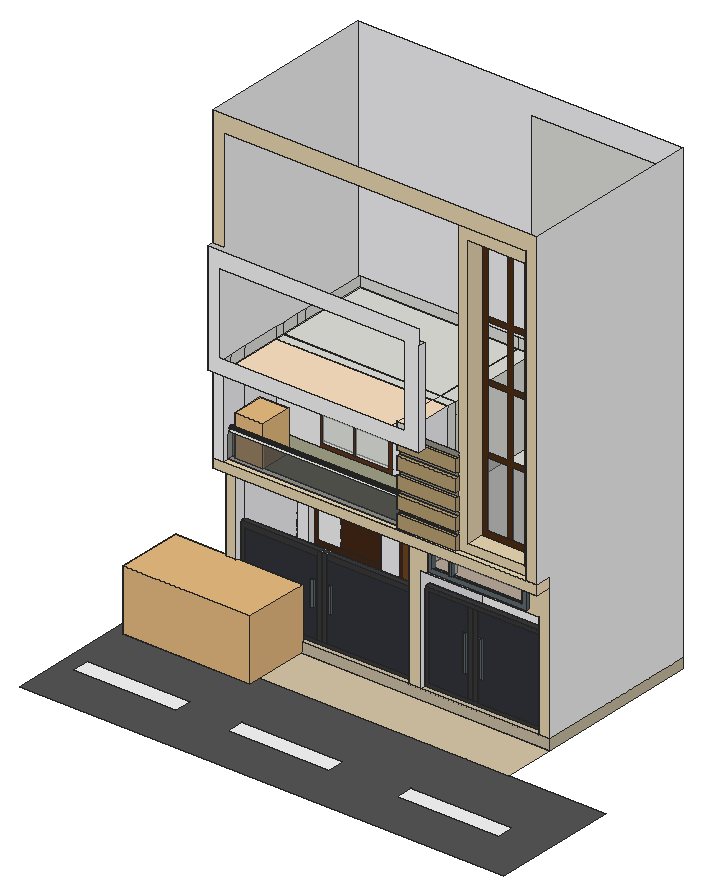
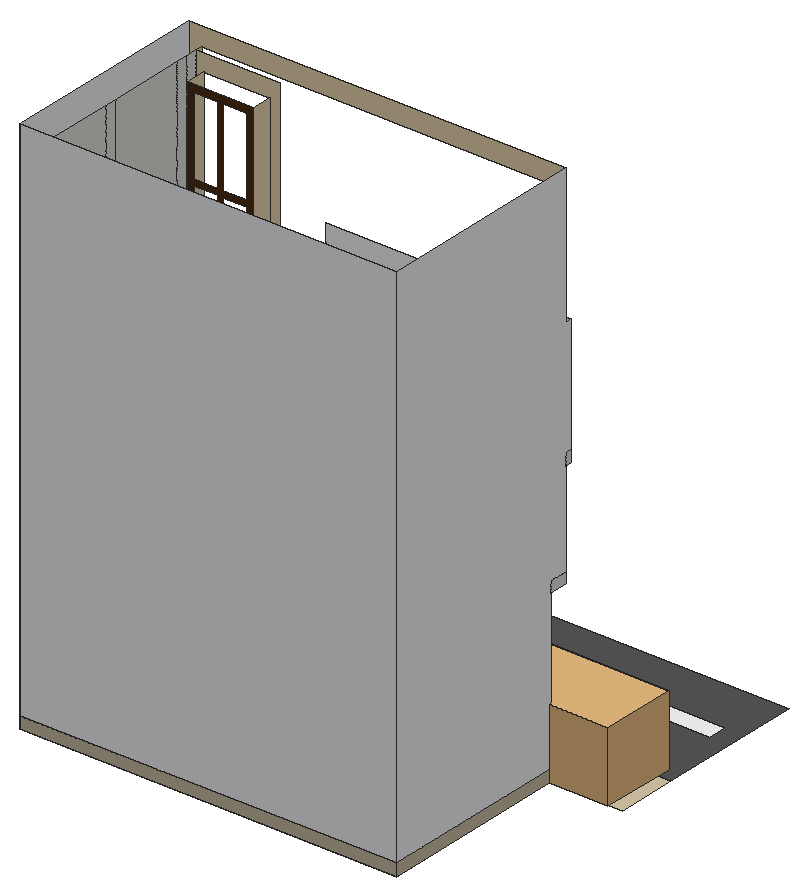
# SketchUp Ruby script. Lengths in inches.
U = 1.inch
M = Sketchup.active_model
def pt(a) = Geom::Point3d.new(a.map { |v| v * U })
def face(e, loops, mat)
  f = e.add_face(loops[0].map { |a| pt(a) })
  loops[1..].each { |l| e.add_face(l.map { |a| pt(a) }).erase! }
  f.material = f.back_material = mat if mat
  f
end
# faces: each face lists its corners as indices into pts; further lists are holes
def faces(e, pts, list, mat = nil) = list.each { |f| face(e, (f[0].is_a?(Array) ? f : [f]).map { |l| l.map { |i| pts[i] } }, mat) }
# xy, xz, yz: faces in a plane at the given z, y or x. An outline is a flat list of corners, or four numbers for a rectangle; further outlines are holes
def ring(l) = l.size == 4 ? [[l[0], l[1]], [l[2], l[1]], [l[2], l[3]], [l[0], l[3]]] : l.each_slice(2).to_a
def flat(e, list, mat, &to3) = list.each { |f| face(e, (f[0].is_a?(Array) ? f : [f]).map { |l| ring(l).map { |u, v| to3.(u, v) } }, mat) }
def xy(e, z, list, mat = nil) = flat(e, list, mat) { |x, y| [x, y, z] }
def xz(e, y, list, mat = nil) = flat(e, list, mat) { |x, z| [x, y, z] }
def yz(e, x, list, mat = nil) = flat(e, list, mat) { |y, z| [x, y, z] }
def lines(e, pts, list) = list.each { |a, b| e.add_line(pt(pts[a]), pt(pts[b])) }
# prism: a flat outline (further loops are holes) pulled along v
def prism(e, loops, v, mat = nil)
  f = face(e, loops, mat); d = Geom::Vector3d.new(v.map { |x| x * U })
  f.pushpull(f.normal.samedirection?(d) ? d.length : -d.length)
end
def box(e, o, s, mat = nil) = prism(e, [[o, [o[0] + s[0], o[1], o[2]], [o[0] + s[0], o[1] + s[1], o[2]], [o[0], o[1] + s[1], o[2]]]], [0, 0, s[2]], mat)
def at(x, y, z, deg = 0) = Geom::Transformation.translation(pt([x, y, z])) * Geom::Transformation.rotation(ORIGIN, Z_AXIS, deg.degrees)
def axes(o, x, y, z) = Geom::Transformation.new([*x, 0, *y, 0, *z, 0, *pt(o).to_a, 1])
def part(name) = M.definitions.add(name)
# library, detail: a bought-in or finely detailed component or shape, given as its bounding box
def library(name, o, s) = part(name).tap { |d| box(d.entities, o, s) }
def detail(e, o, s) = box(e.add_group.entities, o, s)
def put(e, d, t, mat = nil) = e.add_instance(d, t).tap { |i| i.material = mat if mat }
def group(e, t, mat = nil) = e.add_group.tap { |g| g.transformation = t; g.material = mat if mat }.entities
root = M.entities
M.materials.add("[0012_Bisque]").color = [255, 228, 196]
M.materials.add("[Blinds Vertical Pattern]").color = [247, 247, 249]
M.materials.add("[Blinds Vertical Pattern]1").color = [245, 245, 247]
M.materials.add("[Carpet Pattern Squares Multi]").color = [138, 129, 101]
M.materials.add("[Color M06]").color = [86, 86, 86]
M.materials.add("[Color M07]").color = [58, 58, 58]
M.materials.add("[Concrete Tile]").color = [203, 190, 164]
M.materials.add("[Fabric Linen]").color = [161, 161, 136]
M.materials.add("[Field Square Tile]").color = [217, 201, 169]
M.materials.add("[Formica Graystone]").color = [149, 146, 135]
M.materials.add("[Formica Laminate Dark]").color = [50, 53, 60]
M.materials.add("[Formica Speckled Grey]").color = [94, 105, 111]
M.materials.add("[Quartz Light Brown]").color = [234, 216, 179]
M.materials.add("[Quartz Light Grey]").color = [251, 251, 252]
M.materials.add("[Translucent Glass Gray]1").color = [68, 68, 68]
M.materials["[Translucent Glass Gray]1"].alpha = 0.5
M.materials.add("[Translucent Glass Gray]2").color = [128, 128, 128]
M.materials["[Translucent Glass Gray]2"].alpha = 0.5
M.materials.add("[Translucent Glass Safety]1").color = [237, 244, 239]
M.materials["[Translucent Glass Safety]1"].alpha = 0.5
M.materials.add("[Wood Bamboo]").color = [79, 46, 19]
M.materials.add("[Wood Cherry Original]").color = [94, 53, 26]
M.materials.add("[Wood Floor Light]").color = [186, 160, 115]
M.materials.add("[Wood Floor Parquet]").color = [112, 68, 30]
M.materials.add("[Wood Veneer 01]").color = [68, 40, 21]
c1 = library("2015 Porsche Macan",[0.14,0.6,0.32],[90.05,184.43,65.58])
c2 = library("chau cay",[-24.34,-109.24,0],[56.46,62.58,79.69])
xy(root,0,[[123.03,353.85,764.83,681.5]])
xy(root,0,[[[0,0,957,250.875],[33.02,92,234.33,126.875],[336.46,92,537.77,126.875],[671.58,92,872.89,126.875]]],"[Color M06]")
xy(root,0,[[0,250.875,764.83,353.85]],"[Field Square Tile]")
xy(root,0,[[33.02,92,234.33,126.875],[336.46,92,537.77,126.875],[671.58,92,872.89,126.875]],"[Quartz Light Grey]")
xy(root,20.125,[[123.03,353.85,123.03,681.5,764.83,681.5,764.83,353.85,743.35,353.85,743.35,660.02,144.51,660.02,144.51,353.85],[484.74,353.85,509.12,504.41],[144.51,364.59,484.74,375.33],[509.12,364.59,743.35,375.33],[509.12,375.33,743.35,504.41],
  [144.51,504.41,743.35,525.85],[144.51,525.85,743.35,660.02]])
xy(root,20.125,[[144.51,375.33,484.74,504.41]],"[Carpet Pattern Squares Multi]")
xy(root,20.125,[[144.51,353.85,484.74,364.59],[509.12,353.85,743.35,364.59]],"[Concrete Tile]")
xy(root,26.25,[[152.57,364.59,294.93,375.33],[294.93,364.59,304.83,375.33],[304.83,364.59,314.73,375.33],[314.73,364.59,476.37,375.33]])
xy(root,27,[[515.75,364.59,593.81,375.33],[593.81,364.59,603.98,375.33],[603.98,364.59,614.15,375.33],[614.15,364.59,736.66,375.33]])
xy(root,71.5625,[[585.06,361.78,591.37,364.59],[617.68,361.78,623.99,364.59]],"[Formica Speckled Grey]")
xy(root,82.64,[[284.34,361.84,290.96,364.59],[318.96,361.84,325.59,364.59]],"[Formica Speckled Grey]")
xy(root,86.22,[[167.79,504.41,310.48,515.91]],"[Blinds Vertical Pattern]1")
xy(root,132.08,[[284.34,361.84,290.96,364.59],[318.96,361.84,325.59,364.59]],"[Formica Speckled Grey]")
xy(root,142.75,[[585.06,361.78,591.37,364.59],[617.68,361.78,623.99,364.59]],"[Formica Speckled Grey]")
xy(root,185.51,[[144.51,364.59,304.83,375.33],[304.83,364.59,314.73,375.33],[314.73,364.59,476.37,375.33],[476.37,364.59,484.74,375.33]],"[Color M07]")
xy(root,189.34,[[603.98,364.59,614.15,375.33]])
xy(root,197.4375,[[509.12,364.59,736.66,375.33],[736.66,364.59,743.35,375.33]],"[Color M07]")
xy(root,228.92,[[509.12,353.85,743.35,504.41]],"[0012_Bisque]")
xy(root,234.04,[[167.79,504.41,310.48,515.91]],"[Blinds Vertical Pattern]1")
xy(root,235.2,[[527.72,348.16,722.47,353.85]],"[Formica Speckled Grey]")
xy(root,243.53,[[569.36,348.16,574.76,353.85],[569.36,353.85,574.76,361.85]])
xy(root,243.53,[[536.05,348.16,569.36,353.85],[574.76,348.16,714.14,353.85]],"[Formica Speckled Grey]")
xy(root,271.06,[[569.36,348.16,574.76,353.85],[569.36,353.85,574.76,361.85]])
xy(root,271.06,[[536.05,348.16,569.36,353.85],[574.76,348.16,714.14,353.85]],"[Formica Speckled Grey]")
xy(root,279.39,[[527.72,348.16,722.47,353.85]],"[Formica Speckled Grey]")
xy(root,288.25,[[484.74,321.91,509.12,353.85],[509.12,321.91,764.83,353.85],[484.74,353.85,509.12,504.41],[509.12,353.85,743.35,504.41],[144.51,504.41,743.35,525.85],
  [144.51,525.85,743.35,660.02]])
xy(root,288.25,[[123.03,321.91,123.03,353.85,144.51,353.85,144.51,504.41,484.74,504.41,484.74,321.91]],"[0012_Bisque]")
xy(root,307.6875,[[123.03,321.91,144.51,353.85],[743.35,321.91,764.83,353.85],[484.74,326.3,600.81,332.93],[144.51,332.93,484.74,343.39],[484.74,332.93,743.35,660.02],
  [144.51,452.16,484.74,470.45],[144.51,470.45,455.26,660.02],[455.26,470.45,484.74,660.02]])
xy(root,307.6875,[[144.51,343.39,484.74,452.16]],"[Fabric Linen]")
xy(root,307.6875,[[144.51,321.91,484.74,332.93],[484.74,321.91,743.35,321.91,743.35,332.93,600.81,332.93,600.81,326.3,484.74,326.3]],"[Quartz Light Brown]")
xy(root,324.17,[[618.4,332.93,730.9,367.24]],"[Quartz Light Brown]")
xy(root,332.625,[[484.74,326.3,600.81,332.93]],"[Wood Floor Light]")
xy(root,342.125,[[484.74,326.3,600.81,332.93]],"[Wood Floor Light]")
xy(root,357.5625,[[144.51,332.93,484.74,343.39]])
xy(root,367.0625,[[484.74,326.3,600.81,332.93]],"[Wood Floor Light]")
xy(root,376.5625,[[484.74,326.3,600.81,332.93]],"[Wood Floor Light]")
xy(root,401.5,[[484.74,326.3,600.81,332.93]],"[Wood Floor Light]")
xy(root,411,[[484.74,326.3,600.81,332.93]],"[Wood Floor Light]")
xy(root,435.9375,[[484.74,326.3,600.81,332.93]],"[Wood Floor Light]")
xy(root,445.4375,[[484.74,326.3,600.81,332.93]],"[Wood Floor Light]")
xy(root,468.25,[[144.51,452.16,455.26,470.45],[455.26,452.16,484.74,470.45],[144.51,470.45,455.26,660.02],[455.26,470.45,484.74,660.02]])
xy(root,468.25,[[123.03,309.6,123.03,321.91,144.51,321.91,144.51,452.16,455.26,452.16,455.26,309.6],[455.26,309.6,455.26,452.16,484.74,452.16,484.74,324.41,541.38,324.41,541.38,309.6]],"[0012_Bisque]")
xy(root,470.375,[[484.74,326.3,600.81,332.93]],"[Wood Floor Light]")
xz(root,309.6,[[[123.03,468.25,541.38,687.5],[144.51,496.8125,513.0625,656.64]]],"[Blinds Vertical Pattern]")
xz(root,321.91,[[123.03,468.25,144.51,488.6875]])
xz(root,321.91,[[123.03,307.6875,144.51,468.25]],"[Blinds Vertical Pattern]")
xz(root,321.91,[[123.03,288.25,764.83,307.6875],[743.35,307.6875,764.83,307.6875,764.83,923.6875,123.03,923.6875,123.03,687.5,144.51,687.5,144.51,890.6875,743.35,890.6875]],"[Quartz Light Brown]")
xz(root,324.41,[[484.74,468.25,484.74,496.8125,513.0625,496.8125,513.0625,656.64,541.38,656.64,541.38,468.25]])
xz(root,326.3,[[484.74,307.6875,600.81,332.625],[484.74,342.125,600.81,367.0625],[484.74,376.5625,600.81,401.5],[484.74,411,600.81,435.9375],[484.74,445.4375,600.81,470.375]],"[Wood Floor Light]")
xz(root,332.93,[[484.74,307.6875,600.81,332.625],[484.74,342.125,600.81,367.0625],[484.74,376.5625,600.81,401.5],[484.74,411,600.81,435.9375],[484.74,445.4375,600.81,470.375]])
xz(root,332.93,[[484.74,332.625,600.81,342.125],[484.74,367.0625,600.81,376.5625],[484.74,401.5,600.81,411],[484.74,435.9375,600.81,445.4375],[484.74,470.375,600.81,479.875]],"[Formica Graystone]")
xz(root,332.93,[[[600.81,307.6875,743.35,890.6875],[618.4,324.17,730.9,861.54]]],"[Quartz Light Brown]")
xz(root,332.93,[[144.51,307.6875,484.74,357.5625]],"[Translucent Glass Gray]1")
xz(root,343.39,[[144.51,307.6875,484.74,357.5625]],"[Translucent Glass Gray]1")
xz(root,348.16,[[[527.72,235.2,722.47,279.39],[536.05,243.53,714.14,271.06]],[569.36,243.53,574.76,271.06]],"[Formica Speckled Grey]")
xz(root,353.85,[[[527.72,235.2,722.47,279.39],[536.05,243.53,714.14,271.06]],[569.36,243.53,574.76,271.06],[123.03,288.25,144.51,307.6875],[743.35,288.25,764.83,307.6875]])
xz(root,353.85,[[123.03,0,764.83,20.125]],"[Concrete Tile]")
xz(root,353.85,[[123.03,20.125,144.51,288.25],[[484.74,20.125,509.12,20.125,509.12,228.92,743.35,228.92,743.35,20.125,764.83,20.125,764.83,288.25,484.74,288.25],[527.72,235.2,722.47,279.39]]],"[Quartz Light Brown]")
xz(root,353.85,[[536.05,243.53,569.36,271.06],[574.76,243.53,714.14,271.06]],"[Translucent Glass Gray]2")
xz(root,361.78,[[585.06,71.5625,591.37,142.75],[617.68,71.5625,623.99,142.75]],"[Formica Speckled Grey]")
xz(root,361.84,[[284.34,82.64,290.96,132.08],[318.96,82.64,325.59,132.08]],"[Formica Speckled Grey]")
xz(root,361.85,[[569.36,243.53,574.76,271.06]])
xz(root,364.59,[[585.06,71.5625,591.37,142.75],[617.68,71.5625,623.99,142.75]])
xz(root,364.59,[[144.51,20.125,484.74,20.125,484.74,185.51,314.73,185.51,314.73,174.95,476.37,174.95,476.37,26.25,152.57,26.25,152.57,174.95,294.93,174.95,294.93,185.51,144.51,185.51],[[509.12,20.125,743.35,197.4375],[515.75,27,736.66,189.34]],[294.93,26.25,304.83,185.51],[304.83,26.25,314.73,185.51],[593.81,27,603.98,189.34],
  [603.98,27,614.15,189.34]],"[Color M07]")
xz(root,364.59,[[[152.57,26.25,294.93,174.95],[284.34,82.64,290.96,132.08]],[[314.73,26.25,476.37,174.95],[318.96,82.64,325.59,132.08]],[[515.75,27,593.81,189.34],[585.06,71.5625,591.37,142.75]],[[614.15,27,736.66,189.34],[617.68,71.5625,623.99,142.75]]],"[Formica Laminate Dark]")
xz(root,367.24,[[630.125,335.89,670.08,465.11],[679.79,335.89,719.18,465.11]],"[Translucent Glass Gray]2")
xz(root,367.24,[[[618.4,324.17,730.9,861.54],[630.125,335.89,719.18,849.82]],[670.08,335.89,679.79,335.89,679.79,465.11,719.18,465.11,719.18,475.62,679.79,475.62,679.79,594.34,719.18,594.34,719.18,604.84,679.79,604.84,679.79,706.4,719.18,706.4,719.18,716.91,679.79,716.91,679.79,849.82,670.08,849.82,670.08,716.91,630.125,716.91,630.125,706.4,670.08,706.4,670.08,604.84,630.125,604.84,630.125,594.34,670.08,594.34,670.08,475.62,630.125,475.62,630.125,465.11,670.08,465.11]],"[Wood Bamboo]")
xz(root,375.33,[[144.51,20.125,144.51,185.51,294.93,185.51,294.93,174.95,152.57,174.95,152.57,26.25,476.37,26.25,476.37,174.95,314.73,174.95,314.73,185.51,484.74,185.51,484.74,20.125],[[509.12,20.125,743.35,197.4375],[515.75,27,736.66,189.34]],[152.57,26.25,294.93,174.95],[294.93,26.25,304.83,185.51],[304.83,26.25,314.73,185.51],
  [314.73,26.25,476.37,174.95],[515.75,27,593.81,189.34],[593.81,27,603.98,189.34],[603.98,27,614.15,189.34],[614.15,27,736.66,189.34]])
xz(root,452.16,[[144.51,307.6875,230.97,307.6875,230.97,451.25,374.53,451.25,374.53,307.6875,484.74,307.6875,484.74,468.25,144.51,468.25]],"[Blinds Vertical Pattern]")
xz(root,452.16,[[237.93,314.65,297.34,444.29],[302.89,314.65,367.58,444.29]],"[Translucent Glass Safety]1")
xz(root,452.16,[[[230.97,307.6875,374.53,451.25],[237.93,314.65,367.58,444.29]],[297.34,314.65,302.89,444.29]],"[Wood Cherry Original]")
xz(root,470.45,[[144.51,307.6875,455.26,468.25],[455.26,307.6875,484.74,468.25]])
xz(root,504.41,[[484.74,20.125,509.12,288.25],[509.12,228.92,743.35,288.25]])
xz(root,504.41,[[509.12,20.125,743.35,228.92]],"[Blinds Vertical Pattern]")
xz(root,504.41,[[[144.51,20.125,345.37,20.125,345.37,232.5625,467.37,232.5625,467.37,20.125,484.74,20.125,484.74,288.25,144.51,288.25],[167.79,86.22,310.48,234.04]]],"[Blinds Vertical Pattern]1")
xz(root,504.41,[[353.53,28.29,459.21,224.4]],"[Wood Floor Parquet]")
xz(root,504.41,[[[345.37,20.125,467.37,232.5625],[353.53,28.29,459.21,224.4]]],"[Wood Veneer 01]")
xz(root,515.91,[[176.27,94.7,222.36,225.56]],"[Blinds Vertical Pattern]")
xz(root,515.91,[[[167.79,86.22,310.48,234.04],[176.27,94.7,302,225.56]],[222.36,94.7,302,225.56]],"[Wood Veneer 01]")
xz(root,525.85,[[144.51,20.125,743.35,288.25]])
xz(root,660.02,[[144.51,20.125,743.35,288.25],[144.51,288.25,743.35,307.6875],[144.51,307.6875,455.26,468.25],[455.26,307.6875,484.74,468.25],[484.74,307.6875,743.35,890.6875],
  [144.51,468.25,455.26,488.6875],[455.26,468.25,484.74,488.6875]])
xz(root,681.5,[[123.03,20.125,764.83,923.6875]],"[Blinds Vertical Pattern]1")
xz(root,681.5,[[123.03,0,764.83,20.125]],"[Concrete Tile]")
yz(root,123.03,[[321.91,288.25,353.85,307.6875],[309.6,468.25,321.91,488.6875]])
yz(root,123.03,[[353.85,20.125,353.85,307.6875,321.91,307.6875,321.91,488.6875,309.6,488.6875,309.6,687.5,321.91,687.5,321.91,923.6875,681.5,923.6875,681.5,20.125]],"[Blinds Vertical Pattern]1")
yz(root,123.03,[[353.85,0,681.5,20.125]],"[Concrete Tile]")
yz(root,144.51,[[364.59,20.125,375.33,185.51],[504.41,20.125,525.85,288.25],[525.85,20.125,660.02,288.25],[353.85,288.25,375.33,307.6875],[375.33,288.25,504.41,307.6875],
  [504.41,288.25,525.85,307.6875],[525.85,288.25,660.02,307.6875],[332.93,307.6875,343.39,357.5625],[452.16,307.6875,470.45,468.25],[470.45,307.6875,660.02,468.25],
  [338.0625,360.22,337.37,360.31,336.72,360.58,336.16,361,335.74,361.5625,335.47,362.21,335.375,362.91,335.47,363.6,335.74,364.25,336.16,364.81,336.72,365.23,337.37,365.5,338.0625,365.59,338.76,365.5,339.41,365.23,339.96,364.81,340.39,364.25,340.66,363.6,340.75,362.91,340.66,362.21,340.39,361.5625,339.96,361,339.41,360.58,338.76,360.31],[321.91,468.25,321.91,488.6875,341.61,488.6875,332.93,468.25],[332.93,468.25,341.61,488.6875,375.33,488.6875,375.33,468.25],[375.33,468.25,452.16,488.6875],[452.16,468.25,470.45,488.6875],
  [470.45,468.25,504.41,488.6875],[504.41,468.25,525.85,488.6875],[525.85,468.25,660.02,488.6875]])
yz(root,144.51,[[353.85,20.125,364.59,20.125,364.59,185.51,375.33,185.51,375.33,288.25,353.85,288.25],[375.33,20.125,504.41,288.25],[[321.91,307.6875,332.93,307.6875,332.93,357.5625,343.39,357.5625,343.39,307.6875,375.33,307.6875,375.33,468.25,321.91,468.25],[338.0625,360.22,337.37,360.31,336.72,360.58,336.16,361,335.74,361.5625,335.47,362.21,335.375,362.91,335.47,363.6,335.74,364.25,336.16,364.81,336.72,365.23,337.37,365.5,338.0625,365.59,338.76,365.5,339.41,365.23,339.96,364.81,340.39,364.25,340.66,363.6,340.75,362.91,340.66,362.21,340.39,361.5625,339.96,361,339.41,360.58,338.76,360.31]],[375.33,307.6875,452.16,468.25]],"[Blinds Vertical Pattern]")
yz(root,152.57,[[364.59,26.25,375.33,174.95]])
yz(root,167.79,[[504.41,86.22,515.91,234.04]],"[Blinds Vertical Pattern]1")
yz(root,284.34,[[361.84,82.64,364.59,132.08]],"[Formica Speckled Grey]")
yz(root,290.96,[[361.84,82.64,364.59,132.08]],"[Formica Speckled Grey]")
yz(root,294.93,[[364.59,26.25,375.33,174.95]])
yz(root,304.83,[[364.59,26.25,375.33,185.51]])
yz(root,310.48,[[504.41,86.22,515.91,234.04]],"[Blinds Vertical Pattern]1")
yz(root,314.73,[[364.59,26.25,375.33,174.95],[364.59,174.95,375.33,185.51]])
yz(root,318.96,[[361.84,82.64,364.59,132.08]],"[Formica Speckled Grey]")
yz(root,325.59,[[361.84,82.64,364.59,132.08]],"[Formica Speckled Grey]")
yz(root,455.26,[[470.45,307.6875,660.02,468.25]])
yz(root,476.37,[[364.59,26.25,375.33,174.95]])
yz(root,484.74,[[364.59,20.125,375.33,185.51],[332.93,307.6875,343.39,357.5625],[452.16,307.6875,470.45,468.25],[470.45,307.6875,660.02,468.25],[324.41,468.25,326.3,468.25,326.3,470.375,332.93,470.375,332.93,479.875,326.3,479.875,326.3,496.8125,324.41,496.8125],
  [326.3,468.25,332.93,470.375]])
yz(root,484.74,[[353.85,20.125,353.85,288.25,504.41,288.25,504.41,20.125,375.33,20.125,375.33,185.51,364.59,185.51,364.59,20.125],[[343.39,307.6875,343.39,357.5625,332.93,357.5625,332.93,468.25,452.16,468.25,452.16,307.6875],[338.0625,360.22,338.76,360.31,339.41,360.58,339.96,361,340.39,361.5625,340.66,362.21,340.75,362.91,340.66,363.6,340.39,364.25,339.96,364.81,339.41,365.23,338.76,365.5,338.0625,365.59,337.37,365.5,336.72,365.23,336.16,364.81,335.74,364.25,335.47,363.6,335.375,362.91,335.47,362.21,335.74,361.5625,336.16,361,336.72,360.58,337.37,360.31]]],"[Blinds Vertical Pattern]")
yz(root,484.74,[[326.3,307.6875,332.93,332.625],[326.3,342.125,332.93,357.5625],[326.3,357.5625,332.93,367.0625],[326.3,376.5625,332.93,401.5],[326.3,411,332.93,435.9375],
  [326.3,445.4375,332.93,468.25]],"[Wood Floor Light]")
yz(root,509.12,[[364.59,20.125,375.33,197.4375]])
yz(root,509.12,[[353.85,20.125,364.59,20.125,364.59,197.4375,375.33,197.4375,375.33,20.125,504.41,20.125,504.41,228.92,353.85,228.92]],"[Blinds Vertical Pattern]")
yz(root,515.75,[[364.59,27,375.33,189.34]])
yz(root,527.72,[[348.16,235.2,353.85,279.39]],"[Formica Speckled Grey]")
yz(root,536.05,[[348.16,243.53,353.85,271.06]],"[Formica Speckled Grey]")
yz(root,541.38,[[309.6,468.25,324.41,656.64]],"[Blinds Vertical Pattern]")
yz(root,569.36,[[353.85,243.53,361.85,271.06]])
yz(root,569.36,[[348.16,243.53,353.85,271.06]],"[Formica Speckled Grey]")
yz(root,574.76,[[353.85,243.53,361.85,271.06]])
yz(root,574.76,[[348.16,243.53,353.85,271.06]],"[Formica Speckled Grey]")
yz(root,585.06,[[361.78,71.5625,364.59,142.75]],"[Formica Speckled Grey]")
yz(root,591.37,[[361.78,71.5625,364.59,142.75]],"[Formica Speckled Grey]")
yz(root,593.81,[[364.59,27,375.33,189.34]])
yz(root,600.81,[[326.3,307.6875,332.93,332.625],[326.3,342.125,332.93,367.0625],[326.3,376.5625,332.93,401.5],[326.3,411,332.93,435.9375],[326.3,445.4375,332.93,470.375]],"[Wood Floor Light]")
yz(root,603.98,[[364.59,27,375.33,189.34]])
yz(root,614.15,[[364.59,27,375.33,189.34]])
yz(root,617.68,[[361.78,71.5625,364.59,142.75]],"[Formica Speckled Grey]")
yz(root,618.4,[[332.93,324.17,367.24,861.54]],"[Quartz Light Brown]")
yz(root,623.99,[[361.78,71.5625,364.59,142.75]],"[Formica Speckled Grey]")
yz(root,714.14,[[348.16,243.53,353.85,271.06]],"[Formica Speckled Grey]")
yz(root,722.47,[[348.16,235.2,353.85,279.39]],"[Formica Speckled Grey]")
yz(root,730.9,[[332.93,324.17,367.24,861.54]],"[Quartz Light Brown]")
yz(root,736.66,[[364.59,27,375.33,189.34]])
yz(root,743.35,[[364.59,20.125,375.33,197.4375],[504.41,20.125,525.85,288.25],[525.85,20.125,660.02,288.25],[375.33,228.92,504.41,288.25],[353.85,288.25,375.33,307.6875],
  [375.33,288.25,504.41,307.6875],[504.41,288.25,525.85,307.6875],[525.85,288.25,660.02,307.6875],[332.93,307.6875,353.85,890.6875],[353.85,307.6875,375.33,890.6875],
  [375.33,307.6875,504.41,890.6875],[504.41,307.6875,525.85,890.6875],[525.85,307.6875,660.02,890.6875]])
yz(root,743.35,[[353.85,20.125,353.85,228.92,375.33,228.92,375.33,197.4375,364.59,197.4375,364.59,20.125],[375.33,20.125,504.41,228.92]],"[Blinds Vertical Pattern]")
yz(root,743.35,[[321.91,307.6875,332.93,890.6875]],"[Quartz Light Brown]")
yz(root,764.83,[[321.91,288.25,353.85,307.6875]],"[0012_Bisque]")
yz(root,764.83,[[353.85,20.125,681.5,20.125,681.5,923.6875,321.91,923.6875,321.91,307.6875,353.85,307.6875]],"[Blinds Vertical Pattern]1")
yz(root,764.83,[[353.85,0,681.5,20.125]],"[Concrete Tile]")
p = [[144.51,337.37,360.31],[144.51,338.0625,360.22],[484.74,338.0625,360.22],[484.74,337.37,360.31],[144.51,338.76,360.31],[484.74,338.76,360.31],
  [144.51,336.72,360.58],[484.74,336.72,360.58],[144.51,339.41,360.58],[484.74,339.41,360.58],[144.51,336.16,361],[484.74,336.16,361],
  [144.51,339.96,361],[484.74,339.96,361],[144.51,335.74,361.5625],[484.74,335.74,361.5625],[144.51,340.39,361.5625],[484.74,340.39,361.5625],
  [144.51,335.47,362.21],[484.74,335.47,362.21],[144.51,340.66,362.21],[484.74,340.66,362.21],[144.51,335.375,362.91],[484.74,335.375,362.91],
  [144.51,340.75,362.91],[484.74,340.75,362.91],[144.51,335.47,363.6],[484.74,335.47,363.6],[144.51,340.66,363.6],[484.74,340.66,363.6],
  [144.51,335.74,364.25],[484.74,335.74,364.25],[144.51,340.39,364.25],[484.74,340.39,364.25],[144.51,336.16,364.81],[484.74,336.16,364.81],
  [144.51,339.96,364.81],[484.74,339.96,364.81],[144.51,336.72,365.23],[484.74,336.72,365.23],[144.51,339.41,365.23],[484.74,339.41,365.23],
  [144.51,337.37,365.5],[484.74,337.37,365.5],[144.51,338.76,365.5],[484.74,338.76,365.5],[144.51,338.0625,365.59],[484.74,338.0625,365.59]]
faces(root,p,[[0,1,2,3],[1,4,5,2],[6,0,3,7],[4,8,9,5],[10,6,7,11],[8,12,13,9],[14,10,11,15],[12,16,17,13],
  [18,14,15,19],[16,20,21,17],[22,18,19,23],[20,24,25,21],[26,22,23,27],[24,28,29,25],[30,26,27,31],[28,32,33,29],
  [34,30,31,35],[32,36,37,33],[38,34,35,39],[36,40,41,37],[42,38,39,43],[40,44,45,41],[46,42,43,47],[44,46,47,45]],"[Quartz Light Brown]")
put(root,c1,axes([273.69,227.46,0],[0.00953,1.42377,0],[-1.36887,0.00916,0],[0,0,1.8328]))
put(root,c2,at(174.52,452.16,307.6875))
